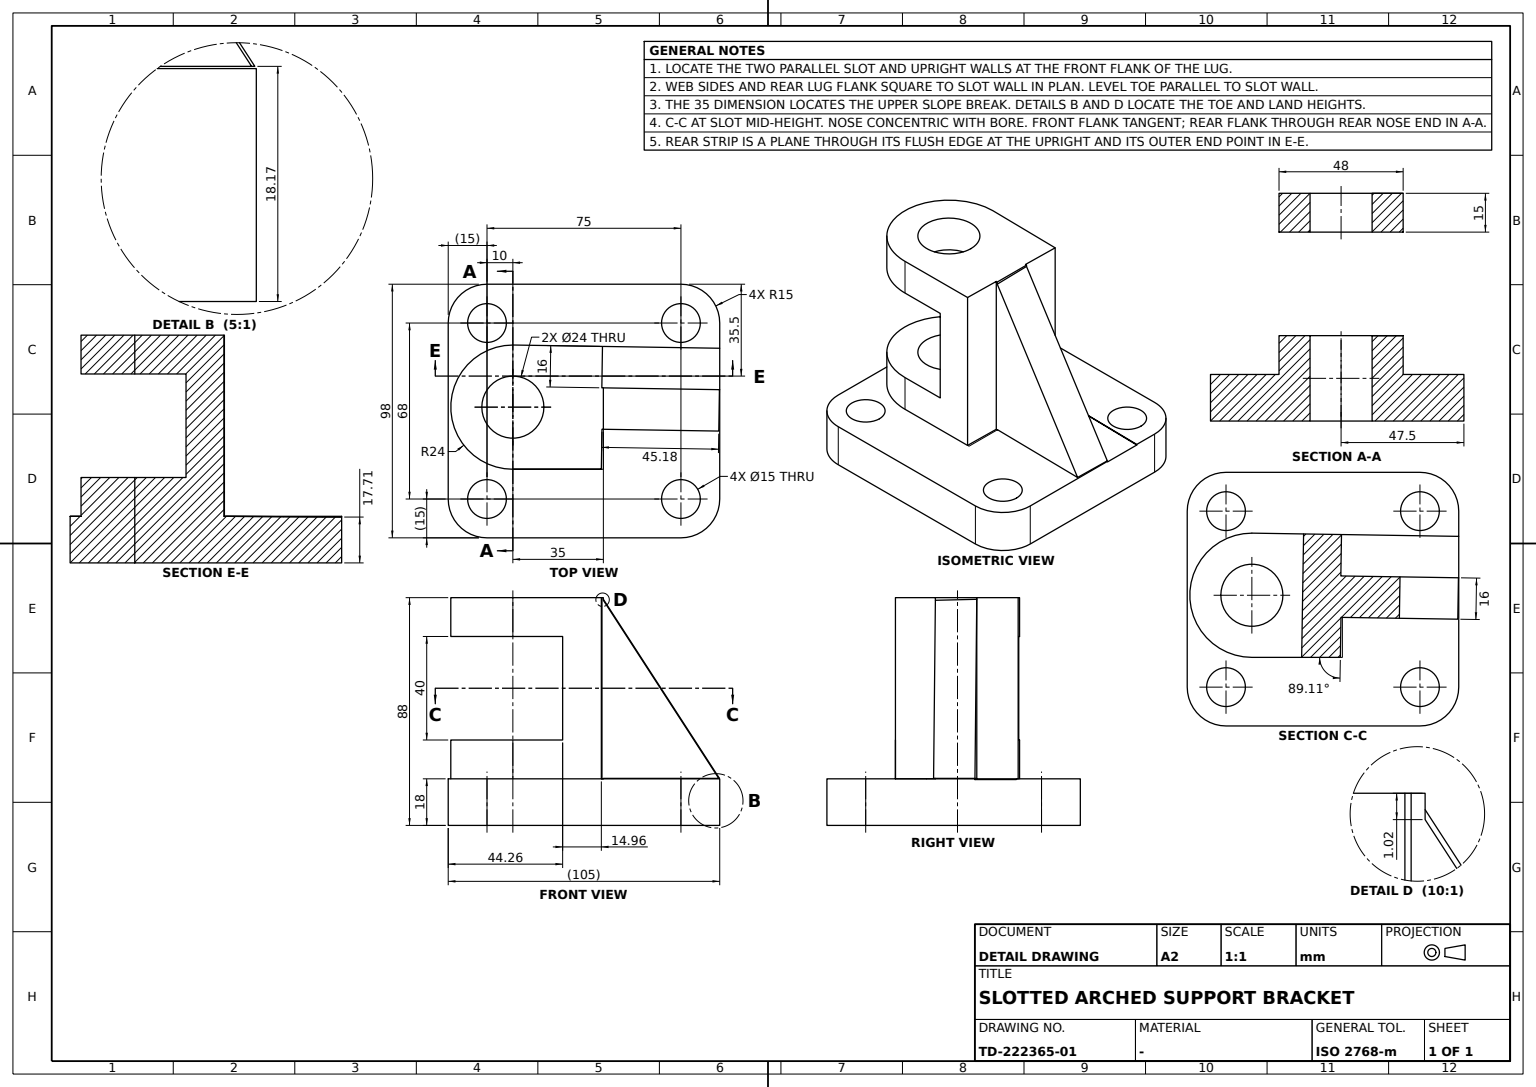
ISO-10303-21;
HEADER;
FILE_DESCRIPTION((''),'2;1');
FILE_NAME('','',(''),(''),'','','');
FILE_SCHEMA(('AUTOMOTIVE_DESIGN'));
ENDSEC;
DATA;
#1=APPLICATION_CONTEXT('');
#2=PRODUCT_CONTEXT('',#1,'mechanical');
#3=PRODUCT('','','',(#2));
#4=PRODUCT_DEFINITION_FORMATION('','',#3);
#5=PRODUCT_DEFINITION_CONTEXT('',#1,'design');
#6=PRODUCT_DEFINITION('','',#4,#5);
#7=PRODUCT_DEFINITION_SHAPE('','',#6);
#8=(LENGTH_UNIT()NAMED_UNIT(*)SI_UNIT(.MILLI.,.METRE.));
#9=(NAMED_UNIT(*)PLANE_ANGLE_UNIT()SI_UNIT($,.RADIAN.));
#10=(NAMED_UNIT(*)SI_UNIT($,.STERADIAN.)SOLID_ANGLE_UNIT());
#11=UNCERTAINTY_MEASURE_WITH_UNIT(LENGTH_MEASURE(0.005),#8,'distance_accuracy_value','');
#12=(GEOMETRIC_REPRESENTATION_CONTEXT(3)GLOBAL_UNCERTAINTY_ASSIGNED_CONTEXT((#11))GLOBAL_UNIT_ASSIGNED_CONTEXT((#8,#9,#10))REPRESENTATION_CONTEXT('',''));
#13=CARTESIAN_POINT('',(60.,57.951587,18.171766));
#14=VERTEX_POINT('',#13);
#15=CARTESIAN_POINT('',(60.,57.951587,18.));
#16=VERTEX_POINT('',#15);
#17=CARTESIAN_POINT('',(60.,57.951587,0.));
#18=DIRECTION('',(0.,0.,-1.));
#19=VECTOR('',#18,1000.);
#20=LINE('',#17,#19);
#21=EDGE_CURVE('',#14,#16,#20,.T.);
#22=ORIENTED_EDGE('',*,*,#21,.F.);
#23=CARTESIAN_POINT('',(60.,41.949637,18.171766));
#24=VERTEX_POINT('',#23);
#25=CARTESIAN_POINT('',(60.,73.953537,18.171766));
#26=DIRECTION('',(0.,-1.,0.));
#27=VECTOR('',#26,1000.);
#28=LINE('',#25,#27);
#29=EDGE_CURVE('',#14,#24,#28,.T.);
#30=ORIENTED_EDGE('',*,*,#29,.T.);
#31=CARTESIAN_POINT('',(60.,41.949637,18.01519));
#32=VERTEX_POINT('',#31);
#33=CARTESIAN_POINT('',(60.,41.949637,18.));
#34=LINE('',#33,#19);
#35=EDGE_CURVE('',#24,#32,#34,.T.);
#36=ORIENTED_EDGE('',*,*,#35,.T.);
#37=CARTESIAN_POINT('',(60.,0.,18.));
#38=DIRECTION('',(0.,1.,0.));
#39=VECTOR('',#38,1000.);
#40=LINE('',#37,#39);
#41=EDGE_CURVE('',#32,#16,#40,.T.);
#42=ORIENTED_EDGE('',*,*,#41,.T.);
#43=EDGE_LOOP('',(#22,#30,#36,#42));
#44=FACE_BOUND('',#43,.T.);
#45=CARTESIAN_POINT('',(60.,26.5,18.));
#46=DIRECTION('',(1.,0.,0.));
#47=AXIS2_PLACEMENT_3D('',#45,#46,#38);
#48=PLANE('',#47);
#49=ADVANCED_FACE('',(#44),#48,.T.);
#50=CARTESIAN_POINT('',(60.,41.949637,88.));
#51=VERTEX_POINT('',#50);
#52=CARTESIAN_POINT('',(59.459336,41.958078,88.));
#53=VERTEX_POINT('',#52);
#54=CARTESIAN_POINT('',(0.669432,42.875979,88.));
#55=DIRECTION('',(-0.999878136,0.015611326,0.));
#56=VECTOR('',#55,1000.);
#57=LINE('',#54,#56);
#58=EDGE_CURVE('',#51,#53,#57,.T.);
#59=ORIENTED_EDGE('',*,*,#58,.F.);
#60=CARTESIAN_POINT('',(60.,57.951587,88.));
#61=VERTEX_POINT('',#60);
#62=CARTESIAN_POINT('',(60.,0.,88.));
#63=LINE('',#62,#39);
#64=EDGE_CURVE('',#51,#61,#63,.T.);
#65=ORIENTED_EDGE('',*,*,#64,.T.);
#66=CARTESIAN_POINT('',(59.408893,57.960816,88.));
#67=VERTEX_POINT('',#66);
#68=CARTESIAN_POINT('',(0.919214,58.874029,88.));
#69=LINE('',#68,#56);
#70=EDGE_CURVE('',#61,#67,#69,.T.);
#71=ORIENTED_EDGE('',*,*,#70,.T.);
#72=CARTESIAN_POINT('',(59.65872,73.961791,88.));
#73=VERTEX_POINT('',#72);
#74=CARTESIAN_POINT('',(59.658674,73.958866,88.));
#75=DIRECTION('',(0.015611326,0.999878136,0.));
#76=VECTOR('',#75,1000.);
#77=LINE('',#74,#76);
#78=EDGE_CURVE('',#67,#73,#77,.T.);
#79=ORIENTED_EDGE('',*,*,#78,.T.);
#80=CARTESIAN_POINT('',(25.,74.5,88.));
#81=VERTEX_POINT('',#80);
#82=CARTESIAN_POINT('',(1.169041,74.875003,88.));
#83=DIRECTION('',(0.999878136,-0.015611326,0.));
#84=VECTOR('',#83,1000.);
#85=LINE('',#82,#84);
#86=EDGE_CURVE('',#81,#73,#85,.T.);
#87=ORIENTED_EDGE('',*,*,#86,.F.);
#88=CARTESIAN_POINT('',(25.,26.5,88.));
#89=VERTEX_POINT('',#88);
#90=CARTESIAN_POINT('',(25.,50.5,88.));
#91=DIRECTION('',(0.,0.,1.));
#92=AXIS2_PLACEMENT_3D('',#90,#91,#46);
#93=CIRCLE('',#92,24.);
#94=EDGE_CURVE('',#81,#89,#93,.T.);
#95=ORIENTED_EDGE('',*,*,#94,.T.);
#96=CARTESIAN_POINT('',(59.217985,26.5,88.));
#97=VERTEX_POINT('',#96);
#98=CARTESIAN_POINT('',(0.,26.5,88.));
#99=VECTOR('',#46,1000.);
#100=LINE('',#98,#99);
#101=EDGE_CURVE('',#89,#97,#100,.T.);
#102=ORIENTED_EDGE('',*,*,#101,.T.);
#103=CARTESIAN_POINT('',(59.209554,25.960028,88.));
#104=LINE('',#103,#76);
#105=EDGE_CURVE('',#97,#53,#104,.T.);
#106=ORIENTED_EDGE('',*,*,#105,.T.);
#107=EDGE_LOOP('',(#59,#65,#71,#79,#87,#95,#102,#106));
#108=FACE_BOUND('',#107,.T.);
#109=CARTESIAN_POINT('',(37.,50.5,88.));
#110=VERTEX_POINT('',#109);
#111=CIRCLE('',#92,12.);
#112=EDGE_CURVE('',#110,#110,#111,.T.);
#113=ORIENTED_EDGE('',*,*,#112,.F.);
#114=EDGE_LOOP('',(#113));
#115=FACE_BOUND('',#114,.T.);
#116=CARTESIAN_POINT('',(0.,0.,88.));
#117=AXIS2_PLACEMENT_3D('',#116,#91,#38);
#118=PLANE('',#117);
#119=ADVANCED_FACE('',(#108,#115),#118,.T.);
#120=CARTESIAN_POINT('',(104.634988,41.252741,18.171766));
#121=VERTEX_POINT('',#120);
#122=CARTESIAN_POINT('',(60.,41.949637,86.980989));
#123=VERTEX_POINT('',#122);
#124=CARTESIAN_POINT('',(82.13498,41.604038,52.857742));
#125=DIRECTION('',(-0.54418844,0.008496539,0.838919991));
#126=VECTOR('',#125,1000.);
#127=LINE('',#124,#126);
#128=EDGE_CURVE('',#121,#123,#127,.T.);
#129=ORIENTED_EDGE('',*,*,#128,.T.);
#130=EDGE_CURVE('',#51,#123,#34,.T.);
#131=ORIENTED_EDGE('',*,*,#130,.F.);
#132=ORIENTED_EDGE('',*,*,#58,.T.);
#133=CARTESIAN_POINT('',(59.459336,41.958078,18.03038));
#134=VERTEX_POINT('',#133);
#135=VECTOR('',#91,1000.);
#136=LINE('',#133,#135);
#137=EDGE_CURVE('',#134,#53,#136,.T.);
#138=ORIENTED_EDGE('',*,*,#137,.F.);
#139=CARTESIAN_POINT('',(105.508072,41.239109,18.03038));
#140=LINE('',#139,#56);
#141=EDGE_CURVE('',#32,#134,#140,.T.);
#142=ORIENTED_EDGE('',*,*,#141,.F.);
#143=ORIENTED_EDGE('',*,*,#35,.F.);
#144=CARTESIAN_POINT('',(0.669432,42.875979,18.171766));
#145=LINE('',#144,#84);
#146=EDGE_CURVE('',#24,#121,#145,.T.);
#147=ORIENTED_EDGE('',*,*,#146,.T.);
#148=EDGE_LOOP('',(#129,#131,#132,#138,#142,#143,#147));
#149=FACE_BOUND('',#148,.T.);
#150=CARTESIAN_POINT('',(0.669432,42.875979,0.));
#151=DIRECTION('',(-0.015611326,-0.999878136,0.));
#152=AXIS2_PLACEMENT_3D('',#150,#151,#83);
#153=PLANE('',#152);
#154=ADVANCED_FACE('',(#149),#153,.T.);
#155=CARTESIAN_POINT('',(15.,0.,0.));
#156=VERTEX_POINT('',#155);
#157=CARTESIAN_POINT('',(15.,0.,18.));
#158=VERTEX_POINT('',#157);
#159=CARTESIAN_POINT('',(15.,0.,9.));
#160=LINE('',#159,#135);
#161=EDGE_CURVE('',#156,#158,#160,.T.);
#162=ORIENTED_EDGE('',*,*,#161,.T.);
#163=CARTESIAN_POINT('',(0.,15.,18.));
#164=VERTEX_POINT('',#163);
#165=CARTESIAN_POINT('',(15.,15.,18.));
#166=AXIS2_PLACEMENT_3D('',#165,#91,#46);
#167=CIRCLE('',#166,15.);
#168=EDGE_CURVE('',#164,#158,#167,.T.);
#169=ORIENTED_EDGE('',*,*,#168,.F.);
#170=CARTESIAN_POINT('',(0.,15.,0.));
#171=VERTEX_POINT('',#170);
#172=CARTESIAN_POINT('',(0.,15.,9.));
#173=LINE('',#172,#135);
#174=EDGE_CURVE('',#171,#164,#173,.T.);
#175=ORIENTED_EDGE('',*,*,#174,.F.);
#176=CARTESIAN_POINT('',(15.,15.,0.));
#177=AXIS2_PLACEMENT_3D('',#176,#91,#46);
#178=CIRCLE('',#177,15.);
#179=EDGE_CURVE('',#171,#156,#178,.T.);
#180=ORIENTED_EDGE('',*,*,#179,.T.);
#181=EDGE_LOOP('',(#162,#169,#175,#180));
#182=FACE_BOUND('',#181,.T.);
#183=CARTESIAN_POINT('',(15.,15.,9.));
#184=AXIS2_PLACEMENT_3D('',#183,#91,#26);
#185=CYLINDRICAL_SURFACE('',#184,15.);
#186=ADVANCED_FACE('',(#182),#185,.T.);
#187=CARTESIAN_POINT('',(105.,57.248992,18.));
#188=VERTEX_POINT('',#187);
#189=CARTESIAN_POINT('',(105.,57.248992,17.713017));
#190=VERTEX_POINT('',#189);
#191=CARTESIAN_POINT('',(105.,57.248992,0.));
#192=LINE('',#191,#19);
#193=EDGE_CURVE('',#188,#190,#192,.T.);
#194=ORIENTED_EDGE('',*,*,#193,.T.);
#195=CARTESIAN_POINT('',(59.408893,57.960816,18.000785));
#196=VERTEX_POINT('',#195);
#197=DIRECTION('',(0.999858223,-0.015611015,-0.006311044));
#198=VECTOR('',#197,1000.);
#199=LINE('',#195,#198);
#200=EDGE_CURVE('',#196,#190,#199,.T.);
#201=ORIENTED_EDGE('',*,*,#200,.F.);
#202=CARTESIAN_POINT('',(59.408893,57.960816,90.075829));
#203=LINE('',#202,#19);
#204=EDGE_CURVE('',#67,#196,#203,.T.);
#205=ORIENTED_EDGE('',*,*,#204,.F.);
#206=ORIENTED_EDGE('',*,*,#70,.F.);
#207=CARTESIAN_POINT('',(60.,57.951587,87.366052));
#208=VERTEX_POINT('',#207);
#209=EDGE_CURVE('',#61,#208,#20,.T.);
#210=ORIENTED_EDGE('',*,*,#209,.T.);
#211=CARTESIAN_POINT('',(104.884769,57.250791,18.171766));
#212=VERTEX_POINT('',#211);
#213=LINE('',#211,#126);
#214=EDGE_CURVE('',#212,#208,#213,.T.);
#215=ORIENTED_EDGE('',*,*,#214,.F.);
#216=CARTESIAN_POINT('',(59.750219,57.955487,18.171766));
#217=LINE('',#216,#84);
#218=EDGE_CURVE('',#14,#212,#217,.T.);
#219=ORIENTED_EDGE('',*,*,#218,.F.);
#220=ORIENTED_EDGE('',*,*,#21,.T.);
#221=CARTESIAN_POINT('',(0.919214,58.874029,18.));
#222=LINE('',#221,#56);
#223=EDGE_CURVE('',#188,#16,#222,.T.);
#224=ORIENTED_EDGE('',*,*,#223,.F.);
#225=EDGE_LOOP('',(#194,#201,#205,#206,#210,#215,#219,#220,#224));
#226=FACE_BOUND('',#225,.T.);
#227=CARTESIAN_POINT('',(0.919214,58.874029,0.));
#228=AXIS2_PLACEMENT_3D('',#227,#75,#55);
#229=PLANE('',#228);
#230=ADVANCED_FACE('',(#226),#229,.T.);
#231=CARTESIAN_POINT('',(59.217985,26.5,18.01519));
#232=VERTEX_POINT('',#231);
#233=CARTESIAN_POINT('',(59.209554,25.960028,18.03038));
#234=LINE('',#233,#76);
#235=EDGE_CURVE('',#232,#134,#234,.T.);
#236=ORIENTED_EDGE('',*,*,#235,.F.);
#237=CARTESIAN_POINT('',(60.,26.5,18.01519));
#238=VERTEX_POINT('',#237);
#239=CARTESIAN_POINT('',(59.217985,26.5,18.03038));
#240=CARTESIAN_POINT('',(59.478657,26.5,18.03038));
#241=CARTESIAN_POINT('',(59.739328,26.5,18.03038));
#242=CARTESIAN_POINT('',(60.,26.5,18.03038));
#243=B_SPLINE_CURVE_WITH_KNOTS('',3,(#239,#240,#241,#242),.UNSPECIFIED.,.F.,.F.,(4,4),(-0.391007418,0.391007168),.UNSPECIFIED.);
#244=EDGE_CURVE('',#238,#232,#243,.F.);
#245=ORIENTED_EDGE('',*,*,#244,.F.);
#246=CARTESIAN_POINT('',(60.,31.649879,18.03038));
#247=CARTESIAN_POINT('',(60.,36.799758,18.03038));
#248=CARTESIAN_POINT('',(60.,41.949637,18.03038));
#249=B_SPLINE_CURVE_WITH_KNOTS('',3,(#242,#246,#247,#248),.UNSPECIFIED.,.F.,.F.,(4,4),(-7.724818179,7.72481821),.UNSPECIFIED.);
#250=EDGE_CURVE('',#32,#238,#249,.F.);
#251=ORIENTED_EDGE('',*,*,#250,.F.);
#252=ORIENTED_EDGE('',*,*,#141,.T.);
#253=EDGE_LOOP('',(#236,#245,#251,#252));
#254=FACE_BOUND('',#253,.T.);
#255=CARTESIAN_POINT('',(105.258291,25.241059,18.03038));
#256=AXIS2_PLACEMENT_3D('',#255,#18,#55);
#257=PLANE('',#256);
#258=ADVANCED_FACE('',(#254),#257,.F.);
#259=ORIENTED_EDGE('',*,*,#204,.T.);
#260=CARTESIAN_POINT('',(59.658674,73.958866,18.000393));
#261=VERTEX_POINT('',#260);
#262=CARTESIAN_POINT('',(59.658674,73.958866,18.000785));
#263=VECTOR('',#151,1000.);
#264=LINE('',#262,#263);
#265=EDGE_CURVE('',#261,#196,#264,.T.);
#266=ORIENTED_EDGE('',*,*,#265,.F.);
#267=CARTESIAN_POINT('',(59.65872,73.961791,18.));
#268=LINE('',#267,#19);
#269=EDGE_CURVE('',#73,#261,#268,.T.);
#270=ORIENTED_EDGE('',*,*,#269,.F.);
#271=ORIENTED_EDGE('',*,*,#78,.F.);
#272=EDGE_LOOP('',(#259,#266,#270,#271));
#273=FACE_BOUND('',#272,.T.);
#274=CARTESIAN_POINT('',(59.658674,73.958866,90.075829));
#275=AXIS2_PLACEMENT_3D('',#274,#55,#18);
#276=PLANE('',#275);
#277=ADVANCED_FACE('',(#273),#276,.F.);
#278=CARTESIAN_POINT('',(25.,74.5,33.));
#279=VERTEX_POINT('',#278);
#280=CARTESIAN_POINT('',(45.001874,74.190631,33.));
#281=VERTEX_POINT('',#280);
#282=CARTESIAN_POINT('',(25.000046,74.502924,33.));
#283=LINE('',#282,#84);
#284=EDGE_CURVE('',#279,#281,#283,.T.);
#285=ORIENTED_EDGE('',*,*,#284,.F.);
#286=CARTESIAN_POINT('',(25.,26.5,33.));
#287=VERTEX_POINT('',#286);
#288=CARTESIAN_POINT('',(25.,50.5,33.));
#289=DIRECTION('',(-1.,0.,0.));
#290=AXIS2_PLACEMENT_3D('',#288,#18,#289);
#291=CIRCLE('',#290,24.);
#292=EDGE_CURVE('',#287,#279,#291,.T.);
#293=ORIENTED_EDGE('',*,*,#292,.F.);
#294=CARTESIAN_POINT('',(44.257269,26.5,33.));
#295=VERTEX_POINT('',#294);
#296=CARTESIAN_POINT('',(0.007311,26.5,33.));
#297=VECTOR('',#289,1000.);
#298=LINE('',#296,#297);
#299=EDGE_CURVE('',#295,#287,#298,.T.);
#300=ORIENTED_EDGE('',*,*,#299,.F.);
#301=CARTESIAN_POINT('',(45.001828,74.187707,33.));
#302=LINE('',#301,#263);
#303=EDGE_CURVE('',#281,#295,#302,.T.);
#304=ORIENTED_EDGE('',*,*,#303,.F.);
#305=EDGE_LOOP('',(#285,#293,#300,#304));
#306=FACE_BOUND('',#305,.T.);
#307=CARTESIAN_POINT('',(13.,50.5,33.));
#308=VERTEX_POINT('',#307);
#309=CIRCLE('',#290,12.);
#310=EDGE_CURVE('',#308,#308,#309,.T.);
#311=ORIENTED_EDGE('',*,*,#310,.T.);
#312=EDGE_LOOP('',(#311));
#313=FACE_BOUND('',#312,.T.);
#314=CARTESIAN_POINT('',(0.007311,74.890217,33.));
#315=AXIS2_PLACEMENT_3D('',#314,#18,#83);
#316=PLANE('',#315);
#317=ADVANCED_FACE('',(#306,#313),#316,.F.);
#318=CARTESIAN_POINT('',(59.217985,26.5,18.));
#319=LINE('',#318,#19);
#320=EDGE_CURVE('',#97,#232,#319,.T.);
#321=ORIENTED_EDGE('',*,*,#320,.T.);
#322=ORIENTED_EDGE('',*,*,#235,.T.);
#323=ORIENTED_EDGE('',*,*,#137,.T.);
#324=ORIENTED_EDGE('',*,*,#105,.F.);
#325=EDGE_LOOP('',(#321,#322,#323,#324));
#326=FACE_BOUND('',#325,.T.);
#327=AXIS2_PLACEMENT_3D('',#233,#55,#91);
#328=PLANE('',#327);
#329=ADVANCED_FACE('',(#326),#328,.F.);
#330=CARTESIAN_POINT('',(22.5,83.,0.));
#331=VERTEX_POINT('',#330);
#332=CARTESIAN_POINT('',(15.,83.,0.));
#333=AXIS2_PLACEMENT_3D('',#332,#91,#46);
#334=CIRCLE('',#333,7.5);
#335=EDGE_CURVE('',#331,#331,#334,.T.);
#336=ORIENTED_EDGE('',*,*,#335,.F.);
#337=EDGE_LOOP('',(#336));
#338=FACE_BOUND('',#337,.T.);
#339=CARTESIAN_POINT('',(22.5,83.,18.));
#340=VERTEX_POINT('',#339);
#341=CARTESIAN_POINT('',(15.,83.,18.));
#342=AXIS2_PLACEMENT_3D('',#341,#91,#46);
#343=CIRCLE('',#342,7.5);
#344=EDGE_CURVE('',#340,#340,#343,.T.);
#345=ORIENTED_EDGE('',*,*,#344,.T.);
#346=EDGE_LOOP('',(#345));
#347=FACE_BOUND('',#346,.T.);
#348=CARTESIAN_POINT('',(15.,83.,17.9));
#349=AXIS2_PLACEMENT_3D('',#348,#18,#46);
#350=CYLINDRICAL_SURFACE('',#349,7.5);
#351=ADVANCED_FACE('',(#338,#347),#350,.F.);
#352=CARTESIAN_POINT('',(25.,26.5,73.));
#353=VERTEX_POINT('',#352);
#354=CARTESIAN_POINT('',(25.,26.5,53.));
#355=LINE('',#354,#135);
#356=EDGE_CURVE('',#353,#89,#355,.T.);
#357=ORIENTED_EDGE('',*,*,#356,.T.);
#358=ORIENTED_EDGE('',*,*,#94,.F.);
#359=CARTESIAN_POINT('',(24.999984,74.5,73.));
#360=VERTEX_POINT('',#359);
#361=CARTESIAN_POINT('',(25.000046,74.502924,73.));
#362=CARTESIAN_POINT('',(25.000046,74.502924,78.));
#363=CARTESIAN_POINT('',(25.000046,74.502924,83.));
#364=CARTESIAN_POINT('',(25.000046,74.502924,88.));
#365=B_SPLINE_CURVE_WITH_KNOTS('',3,(#361,#362,#363,#364),.UNSPECIFIED.,.F.,.F.,(4,4),(0.,1.),.UNSPECIFIED.);
#366=EDGE_CURVE('',#360,#81,#365,.T.);
#367=ORIENTED_EDGE('',*,*,#366,.F.);
#368=CARTESIAN_POINT('',(25.,50.5,73.));
#369=AXIS2_PLACEMENT_3D('',#368,#91,#46);
#370=CIRCLE('',#369,24.);
#371=EDGE_CURVE('',#360,#353,#370,.T.);
#372=ORIENTED_EDGE('',*,*,#371,.T.);
#373=EDGE_LOOP('',(#357,#358,#367,#372));
#374=FACE_BOUND('',#373,.T.);
#375=CARTESIAN_POINT('',(25.,50.5,53.));
#376=AXIS2_PLACEMENT_3D('',#375,#91,#38);
#377=CYLINDRICAL_SURFACE('',#376,24.);
#378=ADVANCED_FACE('',(#374),#377,.T.);
#379=CARTESIAN_POINT('',(60.,24.84998,86.569512));
#380=DIRECTION('',(0.,-0.999710601,-0.024056498));
#381=VECTOR('',#380,1000.);
#382=LINE('',#379,#381);
#383=EDGE_CURVE('',#208,#123,#382,.T.);
#384=ORIENTED_EDGE('',*,*,#383,.F.);
#385=ORIENTED_EDGE('',*,*,#209,.F.);
#386=ORIENTED_EDGE('',*,*,#64,.F.);
#387=ORIENTED_EDGE('',*,*,#130,.T.);
#388=EDGE_LOOP('',(#384,#385,#386,#387));
#389=FACE_BOUND('',#388,.T.);
#390=ADVANCED_FACE('',(#389),#48,.T.);
#391=CARTESIAN_POINT('',(90.,98.,18.));
#392=VERTEX_POINT('',#391);
#393=CARTESIAN_POINT('',(15.,98.,18.));
#394=VERTEX_POINT('',#393);
#395=CARTESIAN_POINT('',(0.,98.,18.));
#396=LINE('',#395,#297);
#397=EDGE_CURVE('',#392,#394,#396,.T.);
#398=ORIENTED_EDGE('',*,*,#397,.F.);
#399=CARTESIAN_POINT('',(90.,98.,0.));
#400=VERTEX_POINT('',#399);
#401=CARTESIAN_POINT('',(90.,98.,9.));
#402=LINE('',#401,#135);
#403=EDGE_CURVE('',#400,#392,#402,.T.);
#404=ORIENTED_EDGE('',*,*,#403,.F.);
#405=CARTESIAN_POINT('',(15.,98.,0.));
#406=VERTEX_POINT('',#405);
#407=CARTESIAN_POINT('',(0.,98.,0.));
#408=LINE('',#407,#297);
#409=EDGE_CURVE('',#400,#406,#408,.T.);
#410=ORIENTED_EDGE('',*,*,#409,.T.);
#411=CARTESIAN_POINT('',(15.,98.,9.));
#412=LINE('',#411,#135);
#413=EDGE_CURVE('',#406,#394,#412,.T.);
#414=ORIENTED_EDGE('',*,*,#413,.T.);
#415=EDGE_LOOP('',(#398,#404,#410,#414));
#416=FACE_BOUND('',#415,.T.);
#417=CARTESIAN_POINT('',(105.,98.,0.));
#418=AXIS2_PLACEMENT_3D('',#417,#38,#289);
#419=PLANE('',#418);
#420=ADVANCED_FACE('',(#416),#419,.T.);
#421=CARTESIAN_POINT('',(90.,0.,0.));
#422=VERTEX_POINT('',#421);
#423=CARTESIAN_POINT('',(90.,0.,18.));
#424=VERTEX_POINT('',#423);
#425=CARTESIAN_POINT('',(90.,0.,9.));
#426=LINE('',#425,#135);
#427=EDGE_CURVE('',#422,#424,#426,.T.);
#428=ORIENTED_EDGE('',*,*,#427,.F.);
#429=CARTESIAN_POINT('',(105.,15.,0.));
#430=VERTEX_POINT('',#429);
#431=CARTESIAN_POINT('',(90.,15.,0.));
#432=AXIS2_PLACEMENT_3D('',#431,#91,#46);
#433=CIRCLE('',#432,15.);
#434=EDGE_CURVE('',#422,#430,#433,.T.);
#435=ORIENTED_EDGE('',*,*,#434,.T.);
#436=CARTESIAN_POINT('',(105.,15.,18.));
#437=VERTEX_POINT('',#436);
#438=CARTESIAN_POINT('',(105.,15.,9.));
#439=LINE('',#438,#135);
#440=EDGE_CURVE('',#430,#437,#439,.T.);
#441=ORIENTED_EDGE('',*,*,#440,.T.);
#442=CARTESIAN_POINT('',(90.,15.,18.));
#443=AXIS2_PLACEMENT_3D('',#442,#91,#46);
#444=CIRCLE('',#443,15.);
#445=EDGE_CURVE('',#424,#437,#444,.T.);
#446=ORIENTED_EDGE('',*,*,#445,.F.);
#447=EDGE_LOOP('',(#428,#435,#441,#446));
#448=FACE_BOUND('',#447,.T.);
#449=CARTESIAN_POINT('',(90.,15.,9.));
#450=AXIS2_PLACEMENT_3D('',#449,#91,#46);
#451=CYLINDRICAL_SURFACE('',#450,15.);
#452=ADVANCED_FACE('',(#448),#451,.T.);
#453=CARTESIAN_POINT('',(37.,50.5,73.));
#454=VERTEX_POINT('',#453);
#455=CIRCLE('',#369,12.);
#456=EDGE_CURVE('',#454,#454,#455,.T.);
#457=ORIENTED_EDGE('',*,*,#456,.F.);
#458=EDGE_LOOP('',(#457));
#459=FACE_BOUND('',#458,.T.);
#460=ORIENTED_EDGE('',*,*,#112,.T.);
#461=EDGE_LOOP('',(#460));
#462=FACE_BOUND('',#461,.T.);
#463=CARTESIAN_POINT('',(25.,50.5,87.9));
#464=AXIS2_PLACEMENT_3D('',#463,#18,#46);
#465=CYLINDRICAL_SURFACE('',#464,12.);
#466=ADVANCED_FACE('',(#459,#462),#465,.F.);
#467=CARTESIAN_POINT('',(25.,26.5,18.));
#468=VERTEX_POINT('',#467);
#469=EDGE_CURVE('',#468,#287,#355,.T.);
#470=ORIENTED_EDGE('',*,*,#469,.T.);
#471=ORIENTED_EDGE('',*,*,#292,.T.);
#472=CARTESIAN_POINT('',(24.999984,74.5,18.));
#473=VERTEX_POINT('',#472);
#474=CARTESIAN_POINT('',(25.000046,74.502924,18.));
#475=CARTESIAN_POINT('',(25.000046,74.502924,23.));
#476=CARTESIAN_POINT('',(25.000046,74.502924,28.));
#477=B_SPLINE_CURVE_WITH_KNOTS('',3,(#474,#475,#476,#282),.UNSPECIFIED.,.F.,.F.,(4,4),(0.,1.),.UNSPECIFIED.);
#478=EDGE_CURVE('',#473,#279,#477,.T.);
#479=ORIENTED_EDGE('',*,*,#478,.F.);
#480=CARTESIAN_POINT('',(25.,50.5,18.));
#481=AXIS2_PLACEMENT_3D('',#480,#91,#46);
#482=CIRCLE('',#481,24.);
#483=EDGE_CURVE('',#473,#468,#482,.T.);
#484=ORIENTED_EDGE('',*,*,#483,.T.);
#485=EDGE_LOOP('',(#470,#471,#479,#484));
#486=FACE_BOUND('',#485,.T.);
#487=ADVANCED_FACE('',(#486),#377,.T.);
#488=CARTESIAN_POINT('',(0.,26.5,18.));
#489=LINE('',#488,#99);
#490=EDGE_CURVE('',#468,#232,#489,.T.);
#491=ORIENTED_EDGE('',*,*,#490,.T.);
#492=ORIENTED_EDGE('',*,*,#320,.F.);
#493=ORIENTED_EDGE('',*,*,#101,.F.);
#494=ORIENTED_EDGE('',*,*,#356,.F.);
#495=CARTESIAN_POINT('',(44.257269,26.5,73.));
#496=VERTEX_POINT('',#495);
#497=LINE('',#352,#297);
#498=EDGE_CURVE('',#496,#353,#497,.T.);
#499=ORIENTED_EDGE('',*,*,#498,.F.);
#500=CARTESIAN_POINT('',(44.257269,26.5,18.));
#501=LINE('',#500,#19);
#502=EDGE_CURVE('',#496,#295,#501,.T.);
#503=ORIENTED_EDGE('',*,*,#502,.T.);
#504=ORIENTED_EDGE('',*,*,#299,.T.);
#505=ORIENTED_EDGE('',*,*,#469,.F.);
#506=EDGE_LOOP('',(#491,#492,#493,#494,#499,#503,#504,#505));
#507=FACE_BOUND('',#506,.T.);
#508=AXIS2_PLACEMENT_3D('',#467,#26,#46);
#509=PLANE('',#508);
#510=ADVANCED_FACE('',(#507),#509,.T.);
#511=CARTESIAN_POINT('',(0.,0.,18.));
#512=LINE('',#511,#99);
#513=EDGE_CURVE('',#158,#424,#512,.T.);
#514=ORIENTED_EDGE('',*,*,#513,.F.);
#515=ORIENTED_EDGE('',*,*,#161,.F.);
#516=CARTESIAN_POINT('',(0.,0.,0.));
#517=LINE('',#516,#99);
#518=EDGE_CURVE('',#156,#422,#517,.T.);
#519=ORIENTED_EDGE('',*,*,#518,.T.);
#520=ORIENTED_EDGE('',*,*,#427,.T.);
#521=EDGE_LOOP('',(#514,#515,#519,#520));
#522=FACE_BOUND('',#521,.T.);
#523=AXIS2_PLACEMENT_3D('',#516,#26,#46);
#524=PLANE('',#523);
#525=ADVANCED_FACE('',(#522),#524,.T.);
#526=CARTESIAN_POINT('',(105.,0.,18.));
#527=LINE('',#526,#27);
#528=EDGE_CURVE('',#188,#437,#527,.T.);
#529=ORIENTED_EDGE('',*,*,#528,.T.);
#530=ORIENTED_EDGE('',*,*,#440,.F.);
#531=CARTESIAN_POINT('',(105.,83.,0.));
#532=VERTEX_POINT('',#531);
#533=CARTESIAN_POINT('',(105.,0.,0.));
#534=LINE('',#533,#27);
#535=EDGE_CURVE('',#532,#430,#534,.T.);
#536=ORIENTED_EDGE('',*,*,#535,.F.);
#537=CARTESIAN_POINT('',(105.,83.,18.));
#538=VERTEX_POINT('',#537);
#539=CARTESIAN_POINT('',(105.,83.,9.));
#540=LINE('',#539,#135);
#541=EDGE_CURVE('',#532,#538,#540,.T.);
#542=ORIENTED_EDGE('',*,*,#541,.T.);
#543=CARTESIAN_POINT('',(105.,73.253867,18.));
#544=VERTEX_POINT('',#543);
#545=EDGE_CURVE('',#538,#544,#527,.T.);
#546=ORIENTED_EDGE('',*,*,#545,.T.);
#547=CARTESIAN_POINT('',(105.,73.253867,17.714594));
#548=VERTEX_POINT('',#547);
#549=LINE('',#543,#19);
#550=EDGE_CURVE('',#544,#548,#549,.T.);
#551=ORIENTED_EDGE('',*,*,#550,.T.);
#552=CARTESIAN_POINT('',(105.,73.958894,17.714663));
#553=DIRECTION('',(0.,0.999999995,0.000098526));
#554=VECTOR('',#553,1000.);
#555=LINE('',#552,#554);
#556=EDGE_CURVE('',#190,#548,#555,.T.);
#557=ORIENTED_EDGE('',*,*,#556,.F.);
#558=ORIENTED_EDGE('',*,*,#193,.F.);
#559=EDGE_LOOP('',(#529,#530,#536,#542,#546,#551,#557,#558));
#560=FACE_BOUND('',#559,.T.);
#561=AXIS2_PLACEMENT_3D('',#417,#289,#26);
#562=PLANE('',#561);
#563=ADVANCED_FACE('',(#560),#562,.F.);
#564=ORIENTED_EDGE('',*,*,#456,.T.);
#565=EDGE_LOOP('',(#564));
#566=FACE_BOUND('',#565,.T.);
#567=ORIENTED_EDGE('',*,*,#371,.F.);
#568=CARTESIAN_POINT('',(45.001874,74.190631,73.));
#569=VERTEX_POINT('',#568);
#570=LINE('',#361,#56);
#571=EDGE_CURVE('',#569,#360,#570,.T.);
#572=ORIENTED_EDGE('',*,*,#571,.F.);
#573=CARTESIAN_POINT('',(45.001828,74.187707,73.));
#574=LINE('',#573,#263);
#575=EDGE_CURVE('',#569,#496,#574,.T.);
#576=ORIENTED_EDGE('',*,*,#575,.T.);
#577=ORIENTED_EDGE('',*,*,#498,.T.);
#578=EDGE_LOOP('',(#567,#572,#576,#577));
#579=FACE_BOUND('',#578,.T.);
#580=AXIS2_PLACEMENT_3D('',#573,#91,#55);
#581=PLANE('',#580);
#582=ADVANCED_FACE('',(#566,#579),#581,.F.);
#583=ORIENTED_EDGE('',*,*,#244,.T.);
#584=ORIENTED_EDGE('',*,*,#490,.F.);
#585=ORIENTED_EDGE('',*,*,#483,.F.);
#586=CARTESIAN_POINT('',(1.169041,74.875003,18.));
#587=LINE('',#586,#84);
#588=EDGE_CURVE('',#473,#261,#587,.T.);
#589=ORIENTED_EDGE('',*,*,#588,.T.);
#590=CARTESIAN_POINT('',(59.783113,73.956923,18.));
#591=VERTEX_POINT('',#590);
#592=CARTESIAN_POINT('',(59.783079,73.956924,18.));
#593=CARTESIAN_POINT('',(59.741612,73.957571,18.000262));
#594=CARTESIAN_POINT('',(59.700144,73.958219,18.000523));
#595=CARTESIAN_POINT('',(59.658677,73.958866,18.000785));
#596=B_SPLINE_CURVE_WITH_KNOTS('',3,(#592,#593,#594,#595),.UNSPECIFIED.,.F.,.F.,(4,4),(0.000002359,0.124422477),.UNSPECIFIED.);
#597=EDGE_CURVE('',#261,#591,#596,.F.);
#598=ORIENTED_EDGE('',*,*,#597,.T.);
#599=CARTESIAN_POINT('',(59.999995,73.953537,17.999315));
#600=VERTEX_POINT('',#599);
#601=CARTESIAN_POINT('',(59.999991,73.953537,17.998631));
#602=CARTESIAN_POINT('',(59.92771,73.954666,17.999087));
#603=CARTESIAN_POINT('',(59.855429,73.955794,17.999543));
#604=CARTESIAN_POINT('',(59.783148,73.956923,18.));
#605=B_SPLINE_CURVE_WITH_KNOTS('',3,(#601,#602,#603,#604),.UNSPECIFIED.,.F.,.F.,(4,4),(45.130812689,45.347686541),.UNSPECIFIED.);
#606=EDGE_CURVE('',#591,#600,#605,.F.);
#607=ORIENTED_EDGE('',*,*,#606,.T.);
#608=LINE('',#474,#56);
#609=EDGE_CURVE('',#544,#600,#608,.T.);
#610=ORIENTED_EDGE('',*,*,#609,.F.);
#611=ORIENTED_EDGE('',*,*,#545,.F.);
#612=CARTESIAN_POINT('',(90.,83.,18.));
#613=AXIS2_PLACEMENT_3D('',#612,#91,#46);
#614=CIRCLE('',#613,15.);
#615=EDGE_CURVE('',#538,#392,#614,.T.);
#616=ORIENTED_EDGE('',*,*,#615,.T.);
#617=ORIENTED_EDGE('',*,*,#397,.T.);
#618=CARTESIAN_POINT('',(0.,83.,18.));
#619=VERTEX_POINT('',#618);
#620=CIRCLE('',#342,15.);
#621=EDGE_CURVE('',#394,#619,#620,.T.);
#622=ORIENTED_EDGE('',*,*,#621,.T.);
#623=LINE('',#511,#39);
#624=EDGE_CURVE('',#164,#619,#623,.T.);
#625=ORIENTED_EDGE('',*,*,#624,.F.);
#626=ORIENTED_EDGE('',*,*,#168,.T.);
#627=ORIENTED_EDGE('',*,*,#513,.T.);
#628=ORIENTED_EDGE('',*,*,#445,.T.);
#629=ORIENTED_EDGE('',*,*,#528,.F.);
#630=ORIENTED_EDGE('',*,*,#223,.T.);
#631=ORIENTED_EDGE('',*,*,#41,.F.);
#632=ORIENTED_EDGE('',*,*,#250,.T.);
#633=EDGE_LOOP('',(#583,#584,#585,#589,#598,#607,#610,#611,#616,#617,#622,#625,#626,#627,#628,#629,#630,#631,#632));
#634=FACE_BOUND('',#633,.T.);
#635=CARTESIAN_POINT('',(97.5,15.,18.));
#636=VERTEX_POINT('',#635);
#637=CIRCLE('',#443,7.5);
#638=EDGE_CURVE('',#636,#636,#637,.T.);
#639=ORIENTED_EDGE('',*,*,#638,.F.);
#640=EDGE_LOOP('',(#639));
#641=FACE_BOUND('',#640,.T.);
#642=CARTESIAN_POINT('',(22.5,15.,18.));
#643=VERTEX_POINT('',#642);
#644=CIRCLE('',#166,7.5);
#645=EDGE_CURVE('',#643,#643,#644,.T.);
#646=ORIENTED_EDGE('',*,*,#645,.F.);
#647=EDGE_LOOP('',(#646));
#648=FACE_BOUND('',#647,.T.);
#649=ORIENTED_EDGE('',*,*,#344,.F.);
#650=EDGE_LOOP('',(#649));
#651=FACE_BOUND('',#650,.T.);
#652=CARTESIAN_POINT('',(97.5,83.,18.));
#653=VERTEX_POINT('',#652);
#654=CIRCLE('',#613,7.5);
#655=EDGE_CURVE('',#653,#653,#654,.T.);
#656=ORIENTED_EDGE('',*,*,#655,.F.);
#657=EDGE_LOOP('',(#656));
#658=FACE_BOUND('',#657,.T.);
#659=AXIS2_PLACEMENT_3D('',#511,#91,#38);
#660=PLANE('',#659);
#661=ADVANCED_FACE('',(#634,#641,#648,#651,#658),#660,.T.);
#662=CARTESIAN_POINT('',(97.5,15.,0.));
#663=VERTEX_POINT('',#662);
#664=CIRCLE('',#432,7.5);
#665=EDGE_CURVE('',#663,#663,#664,.T.);
#666=ORIENTED_EDGE('',*,*,#665,.F.);
#667=EDGE_LOOP('',(#666));
#668=FACE_BOUND('',#667,.T.);
#669=ORIENTED_EDGE('',*,*,#638,.T.);
#670=EDGE_LOOP('',(#669));
#671=FACE_BOUND('',#670,.T.);
#672=CARTESIAN_POINT('',(90.,15.,17.9));
#673=AXIS2_PLACEMENT_3D('',#672,#18,#46);
#674=CYLINDRICAL_SURFACE('',#673,7.5);
#675=ADVANCED_FACE('',(#668,#671),#674,.F.);
#676=ORIENTED_EDGE('',*,*,#146,.F.);
#677=ORIENTED_EDGE('',*,*,#29,.F.);
#678=ORIENTED_EDGE('',*,*,#218,.T.);
#679=CARTESIAN_POINT('',(105.13455,73.248841,18.171766));
#680=LINE('',#679,#263);
#681=EDGE_CURVE('',#212,#121,#680,.T.);
#682=ORIENTED_EDGE('',*,*,#681,.T.);
#683=EDGE_LOOP('',(#676,#677,#678,#682));
#684=FACE_BOUND('',#683,.T.);
#685=AXIS2_PLACEMENT_3D('',#25,#18,#83);
#686=PLANE('',#685);
#687=ADVANCED_FACE('',(#684),#686,.T.);
#688=CARTESIAN_POINT('',(0.,83.,0.));
#689=VERTEX_POINT('',#688);
#690=CARTESIAN_POINT('',(0.,83.,9.));
#691=LINE('',#690,#135);
#692=EDGE_CURVE('',#689,#619,#691,.T.);
#693=ORIENTED_EDGE('',*,*,#692,.F.);
#694=LINE('',#516,#39);
#695=EDGE_CURVE('',#171,#689,#694,.T.);
#696=ORIENTED_EDGE('',*,*,#695,.F.);
#697=ORIENTED_EDGE('',*,*,#174,.T.);
#698=ORIENTED_EDGE('',*,*,#624,.T.);
#699=EDGE_LOOP('',(#693,#696,#697,#698));
#700=FACE_BOUND('',#699,.T.);
#701=AXIS2_PLACEMENT_3D('',#516,#46,#38);
#702=PLANE('',#701);
#703=ADVANCED_FACE('',(#700),#702,.F.);
#704=ORIENTED_EDGE('',*,*,#541,.F.);
#705=CARTESIAN_POINT('',(90.,83.,0.));
#706=AXIS2_PLACEMENT_3D('',#705,#91,#46);
#707=CIRCLE('',#706,15.);
#708=EDGE_CURVE('',#532,#400,#707,.T.);
#709=ORIENTED_EDGE('',*,*,#708,.T.);
#710=ORIENTED_EDGE('',*,*,#403,.T.);
#711=ORIENTED_EDGE('',*,*,#615,.F.);
#712=EDGE_LOOP('',(#704,#709,#710,#711));
#713=FACE_BOUND('',#712,.T.);
#714=CARTESIAN_POINT('',(90.,83.,9.));
#715=AXIS2_PLACEMENT_3D('',#714,#91,#38);
#716=CYLINDRICAL_SURFACE('',#715,15.);
#717=ADVANCED_FACE('',(#713),#716,.T.);
#718=ORIENTED_EDGE('',*,*,#645,.T.);
#719=EDGE_LOOP('',(#718));
#720=FACE_BOUND('',#719,.T.);
#721=CARTESIAN_POINT('',(22.5,15.,0.));
#722=VERTEX_POINT('',#721);
#723=CIRCLE('',#177,7.5);
#724=EDGE_CURVE('',#722,#722,#723,.T.);
#725=ORIENTED_EDGE('',*,*,#724,.F.);
#726=EDGE_LOOP('',(#725));
#727=FACE_BOUND('',#726,.T.);
#728=CARTESIAN_POINT('',(15.,15.,17.9));
#729=AXIS2_PLACEMENT_3D('',#728,#18,#46);
#730=CYLINDRICAL_SURFACE('',#729,7.5);
#731=ADVANCED_FACE('',(#720,#727),#730,.F.);
#732=CARTESIAN_POINT('',(37.,50.5,0.));
#733=VERTEX_POINT('',#732);
#734=CARTESIAN_POINT('',(25.,50.5,0.));
#735=AXIS2_PLACEMENT_3D('',#734,#91,#46);
#736=CIRCLE('',#735,12.);
#737=EDGE_CURVE('',#733,#733,#736,.T.);
#738=ORIENTED_EDGE('',*,*,#737,.T.);
#739=EDGE_LOOP('',(#738));
#740=FACE_BOUND('',#739,.T.);
#741=ORIENTED_EDGE('',*,*,#665,.T.);
#742=EDGE_LOOP('',(#741));
#743=FACE_BOUND('',#742,.T.);
#744=ORIENTED_EDGE('',*,*,#724,.T.);
#745=EDGE_LOOP('',(#744));
#746=FACE_BOUND('',#745,.T.);
#747=ORIENTED_EDGE('',*,*,#335,.T.);
#748=EDGE_LOOP('',(#747));
#749=FACE_BOUND('',#748,.T.);
#750=ORIENTED_EDGE('',*,*,#695,.T.);
#751=CIRCLE('',#333,15.);
#752=EDGE_CURVE('',#406,#689,#751,.T.);
#753=ORIENTED_EDGE('',*,*,#752,.F.);
#754=ORIENTED_EDGE('',*,*,#409,.F.);
#755=ORIENTED_EDGE('',*,*,#708,.F.);
#756=ORIENTED_EDGE('',*,*,#535,.T.);
#757=ORIENTED_EDGE('',*,*,#434,.F.);
#758=ORIENTED_EDGE('',*,*,#518,.F.);
#759=ORIENTED_EDGE('',*,*,#179,.F.);
#760=EDGE_LOOP('',(#750,#753,#754,#755,#756,#757,#758,#759));
#761=FACE_BOUND('',#760,.T.);
#762=CARTESIAN_POINT('',(97.5,83.,0.));
#763=VERTEX_POINT('',#762);
#764=CIRCLE('',#706,7.5);
#765=EDGE_CURVE('',#763,#763,#764,.T.);
#766=ORIENTED_EDGE('',*,*,#765,.T.);
#767=EDGE_LOOP('',(#766));
#768=FACE_BOUND('',#767,.T.);
#769=AXIS2_PLACEMENT_3D('',#516,#91,#38);
#770=PLANE('',#769);
#771=ADVANCED_FACE('',(#740,#743,#746,#749,#761,#768),#770,.F.);
#772=ORIENTED_EDGE('',*,*,#609,.T.);
#773=CARTESIAN_POINT('',(25.001431,74.502903,18.21954));
#774=LINE('',#773,#198);
#775=EDGE_CURVE('',#600,#548,#774,.T.);
#776=ORIENTED_EDGE('',*,*,#775,.T.);
#777=ORIENTED_EDGE('',*,*,#550,.F.);
#778=EDGE_LOOP('',(#772,#776,#777));
#779=FACE_BOUND('',#778,.T.);
#780=AXIS2_PLACEMENT_3D('',#474,#151,#83);
#781=PLANE('',#780);
#782=ADVANCED_FACE('',(#779),#781,.T.);
#783=ORIENTED_EDGE('',*,*,#681,.F.);
#784=ORIENTED_EDGE('',*,*,#214,.T.);
#785=ORIENTED_EDGE('',*,*,#383,.T.);
#786=ORIENTED_EDGE('',*,*,#128,.F.);
#787=EDGE_LOOP('',(#783,#784,#785,#786));
#788=FACE_BOUND('',#787,.T.);
#789=DIRECTION('',(0.838817756,-0.013096654,0.544254765));
#790=AXIS2_PLACEMENT_3D('',#679,#789,#125);
#791=PLANE('',#790);
#792=ADVANCED_FACE('',(#788),#791,.T.);
#793=ORIENTED_EDGE('',*,*,#737,.F.);
#794=EDGE_LOOP('',(#793));
#795=FACE_BOUND('',#794,.T.);
#796=ORIENTED_EDGE('',*,*,#310,.F.);
#797=EDGE_LOOP('',(#796));
#798=FACE_BOUND('',#797,.T.);
#799=ADVANCED_FACE('',(#795,#798),#465,.F.);
#800=ORIENTED_EDGE('',*,*,#303,.T.);
#801=ORIENTED_EDGE('',*,*,#502,.F.);
#802=ORIENTED_EDGE('',*,*,#575,.F.);
#803=CARTESIAN_POINT('',(45.001874,74.190631,18.));
#804=LINE('',#803,#19);
#805=EDGE_CURVE('',#569,#281,#804,.T.);
#806=ORIENTED_EDGE('',*,*,#805,.T.);
#807=EDGE_LOOP('',(#800,#801,#802,#806));
#808=FACE_BOUND('',#807,.T.);
#809=AXIS2_PLACEMENT_3D('',#573,#55,#18);
#810=PLANE('',#809);
#811=ADVANCED_FACE('',(#808),#810,.T.);
#812=ORIENTED_EDGE('',*,*,#200,.T.);
#813=ORIENTED_EDGE('',*,*,#556,.T.);
#814=ORIENTED_EDGE('',*,*,#775,.F.);
#815=ORIENTED_EDGE('',*,*,#606,.F.);
#816=ORIENTED_EDGE('',*,*,#597,.F.);
#817=ORIENTED_EDGE('',*,*,#265,.T.);
#818=EDGE_LOOP('',(#812,#813,#814,#815,#816,#817));
#819=FACE_BOUND('',#818,.T.);
#820=DIRECTION('',(-0.006310274,0.000098524,-0.999980085));
#821=AXIS2_PLACEMENT_3D('',#262,#820,#197);
#822=PLANE('',#821);
#823=ADVANCED_FACE('',(#819),#822,.F.);
#824=ORIENTED_EDGE('',*,*,#655,.T.);
#825=EDGE_LOOP('',(#824));
#826=FACE_BOUND('',#825,.T.);
#827=ORIENTED_EDGE('',*,*,#765,.F.);
#828=EDGE_LOOP('',(#827));
#829=FACE_BOUND('',#828,.T.);
#830=CARTESIAN_POINT('',(90.,83.,17.9));
#831=AXIS2_PLACEMENT_3D('',#830,#18,#46);
#832=CYLINDRICAL_SURFACE('',#831,7.5);
#833=ADVANCED_FACE('',(#826,#829),#832,.F.);
#834=ORIENTED_EDGE('',*,*,#752,.T.);
#835=ORIENTED_EDGE('',*,*,#692,.T.);
#836=ORIENTED_EDGE('',*,*,#621,.F.);
#837=ORIENTED_EDGE('',*,*,#413,.F.);
#838=EDGE_LOOP('',(#834,#835,#836,#837));
#839=FACE_BOUND('',#838,.T.);
#840=CARTESIAN_POINT('',(15.,83.,9.));
#841=AXIS2_PLACEMENT_3D('',#840,#91,#289);
#842=CYLINDRICAL_SURFACE('',#841,15.);
#843=ADVANCED_FACE('',(#839),#842,.T.);
#844=ORIENTED_EDGE('',*,*,#366,.T.);
#845=ORIENTED_EDGE('',*,*,#86,.T.);
#846=ORIENTED_EDGE('',*,*,#269,.T.);
#847=ORIENTED_EDGE('',*,*,#588,.F.);
#848=ORIENTED_EDGE('',*,*,#478,.T.);
#849=ORIENTED_EDGE('',*,*,#284,.T.);
#850=ORIENTED_EDGE('',*,*,#805,.F.);
#851=ORIENTED_EDGE('',*,*,#571,.T.);
#852=EDGE_LOOP('',(#844,#845,#846,#847,#848,#849,#850,#851));
#853=FACE_BOUND('',#852,.T.);
#854=ADVANCED_FACE('',(#853),#781,.F.);
#855=CLOSED_SHELL('',(#49,#119,#154,#186,#230,#258,#277,#317,#329,#351,#378,#390,#420,#452,#466,#487,#510,#525,#563,#582,#661,#675,#687,#703,#717,#731,#771,#782,#792,#799,#811,#823,#833,#843,#854));
#856=MANIFOLD_SOLID_BREP('',#855);
#857=ADVANCED_BREP_SHAPE_REPRESENTATION('',(#856),#12);
#858=SHAPE_DEFINITION_REPRESENTATION(#7,#857);
ENDSEC;
END-ISO-10303-21;
